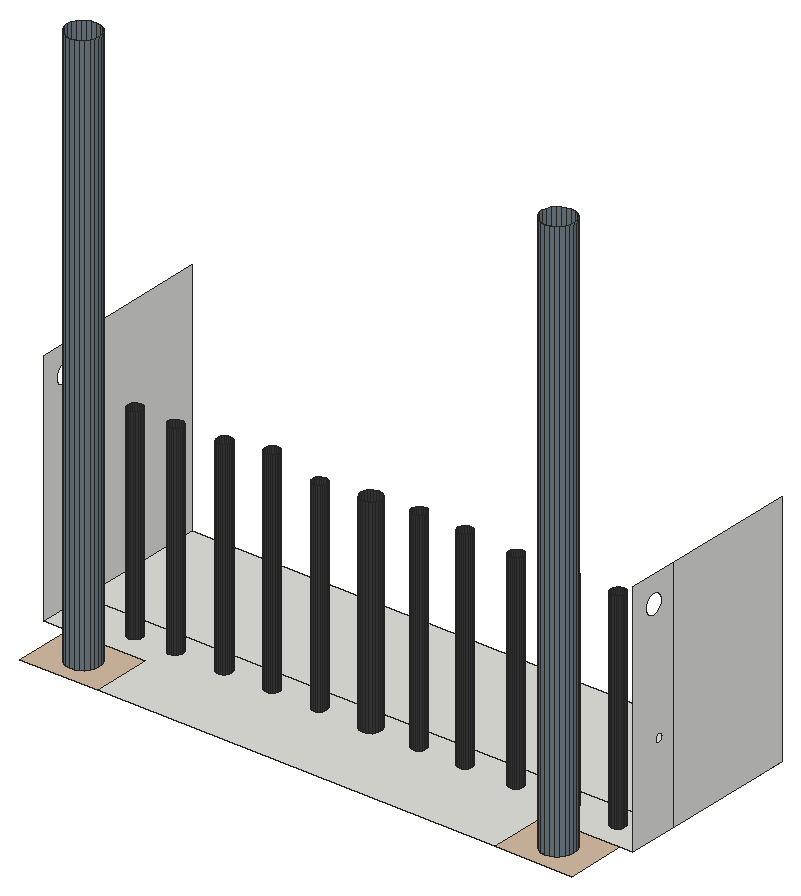
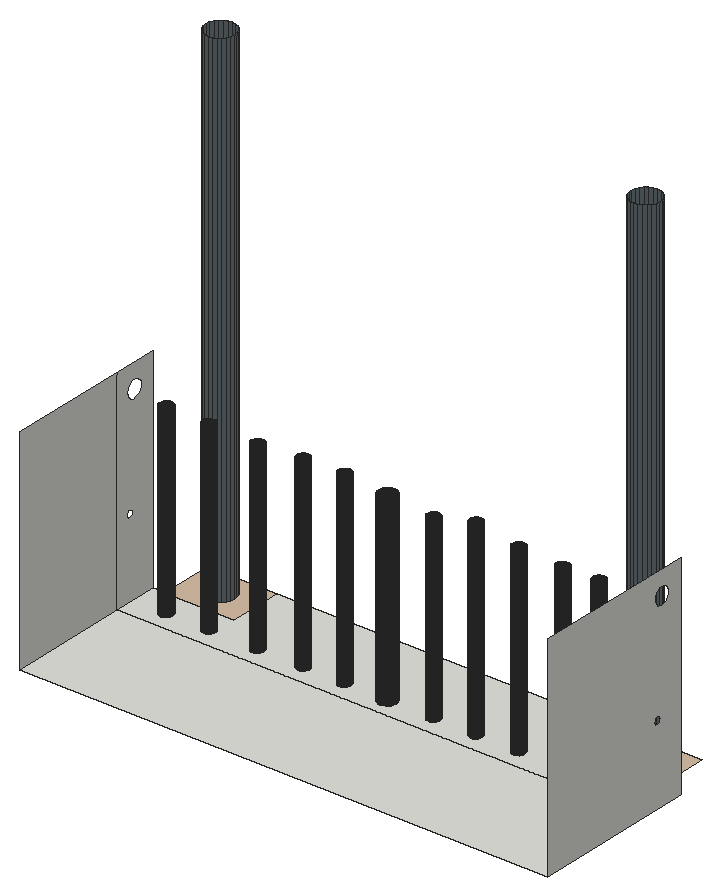
# SketchUp Ruby script. Lengths in inches.
U = 1.inch
M = Sketchup.active_model
def pt(a) = Geom::Point3d.new(a.map { |v| v * U })
def face(e, loops, mat)
  f = e.add_face(loops[0].map { |a| pt(a) })
  loops[1..].each { |l| e.add_face(l.map { |a| pt(a) }).erase! }
  f.material = f.back_material = mat if mat
  f
end
# faces: each face lists its corners as indices into pts; further lists are holes
def faces(e, pts, list, mat = nil) = list.each { |f| face(e, (f[0].is_a?(Array) ? f : [f]).map { |l| l.map { |i| pts[i] } }, mat) }
# xy, xz, yz: faces in a plane at the given z, y or x. An outline is a flat list of corners, or four numbers for a rectangle; further outlines are holes
def ring(l) = l.size == 4 ? [[l[0], l[1]], [l[2], l[1]], [l[2], l[3]], [l[0], l[3]]] : l.each_slice(2).to_a
def flat(e, list, mat, &to3) = list.each { |f| face(e, (f[0].is_a?(Array) ? f : [f]).map { |l| ring(l).map { |u, v| to3.(u, v) } }, mat) }
def xy(e, z, list, mat = nil) = flat(e, list, mat) { |x, y| [x, y, z] }
def xz(e, y, list, mat = nil) = flat(e, list, mat) { |x, z| [x, y, z] }
def yz(e, x, list, mat = nil) = flat(e, list, mat) { |y, z| [x, y, z] }
def lines(e, pts, list) = list.each { |a, b| e.add_line(pt(pts[a]), pt(pts[b])) }
# prism: a flat outline (further loops are holes) pulled along v
def prism(e, loops, v, mat = nil)
  f = face(e, loops, mat); d = Geom::Vector3d.new(v.map { |x| x * U })
  f.pushpull(f.normal.samedirection?(d) ? d.length : -d.length)
end
def box(e, o, s, mat = nil) = prism(e, [[o, [o[0] + s[0], o[1], o[2]], [o[0] + s[0], o[1] + s[1], o[2]], [o[0], o[1] + s[1], o[2]]]], [0, 0, s[2]], mat)
def at(x, y, z, deg = 0) = Geom::Transformation.translation(pt([x, y, z])) * Geom::Transformation.rotation(ORIGIN, Z_AXIS, deg.degrees)
def axes(o, x, y, z) = Geom::Transformation.new([*x, 0, *y, 0, *z, 0, *pt(o).to_a, 1])
def part(name) = M.definitions.add(name)
# library, detail: a bought-in or finely detailed component or shape, given as its bounding box
def library(name, o, s) = part(name).tap { |d| box(d.entities, o, s) }
def detail(e, o, s) = box(e.add_group.entities, o, s)
def put(e, d, t, mat = nil) = e.add_instance(d, t).tap { |i| i.material = mat if mat }
def group(e, t, mat = nil) = e.add_group.tap { |g| g.transformation = t; g.material = mat if mat }.entities
root = M.entities
M.materials.add("[Color M07]").color = [58, 58, 58]
M.materials.add("[Formica Laminate Light]").color = [213, 189, 164]
M.materials.add("[Formica Speckled Grey]").color = [112, 125, 132]
xy(root,162.85,[[[59.48,81.92,111.73,81.92,111.73,89.73,123.57,89.73,123.57,96.35,46.18,96.35,46.18,89.73,59.48,89.73],[86.23,92.1,85.89,92.15,85.57,92.28,85.3,92.48,85.09,92.76,84.96,93.07,84.92,93.41,84.96,93.75,85.09,94.07,85.3,94.34,85.57,94.55,85.89,94.68,86.23,94.73,86.57,94.68,86.89,94.55,87.16,94.34,87.37,94.07,87.5,93.75,87.54,93.41,87.5,93.07,87.37,92.76,87.16,92.48,86.89,92.28,86.57,92.15],[92.58,92.43,92.34,92.46,92.11,92.55,91.92,92.7,91.77,92.9,91.67,93.125,91.64,93.37,91.67,93.61,91.77,93.83,91.92,94.03,92.11,94.18,92.34,94.27,92.58,94.3,92.82,94.27,93.05,94.18,93.24,94.03,93.39,93.83,93.48,93.61,93.52,93.37,93.48,93.125,93.39,92.9,93.24,92.7,93.05,92.55,92.82,92.46],[98.64,92.43,98.4,92.46,98.17,92.55,97.98,92.7,97.83,92.9,97.74,93.125,97.7,93.37,97.74,93.61,97.83,93.83,97.98,94.03,98.17,94.18,98.4,94.27,98.64,94.3,98.88,94.27,99.11,94.18,99.3,94.03,99.45,93.83,99.55,93.61,99.58,93.37,99.55,93.125,99.45,92.9,99.3,92.7,99.11,92.55,98.88,92.46],[105.33,92.43,105.09,92.46,104.86,92.55,104.67,92.7,104.52,92.9,104.42,93.125,104.39,93.37,104.42,93.61,104.52,93.83,104.67,94.03,104.86,94.18,105.09,94.27,105.33,94.3,105.57,94.27,105.8,94.18,105.99,94.03,106.14,93.83,106.23,93.61,106.27,93.37,106.23,93.125,106.14,92.9,105.99,92.7,105.8,92.55,105.57,92.46],[112.45,92.43,112.21,92.46,111.99,92.55,111.79,92.7,111.64,92.9,111.55,93.125,111.52,93.37,111.55,93.61,111.64,93.83,111.79,94.03,111.99,94.18,112.21,94.27,112.45,94.3,112.7,94.27,112.92,94.18,113.12,94.03,113.27,93.83,113.36,93.61,113.39,93.37,113.36,93.125,113.27,92.9,113.12,92.7,112.92,92.55,112.7,92.46],[79.52,92.43,79.27,92.46,79.05,92.55,78.85,92.7,78.7,92.9,78.61,93.125,78.58,93.37,78.61,93.61,78.7,93.83,78.85,94.03,79.05,94.18,79.27,94.27,79.52,94.3,79.76,94.27,79.99,94.18,80.18,94.03,80.33,93.83,80.42,93.61,80.45,93.37,80.42,93.125,80.33,92.9,80.18,92.7,79.99,92.55,79.76,92.46],[49.7,92.43,49.46,92.46,49.24,92.55,49.04,92.7,48.89,92.9,48.8,93.125,48.77,93.37,48.8,93.61,48.89,93.83,49.04,94.03,49.24,94.18,49.46,94.27,49.7,94.3,49.95,94.27,50.17,94.18,50.37,94.03,50.52,93.83,50.61,93.61,50.64,93.37,50.61,93.125,50.52,92.9,50.37,92.7,50.17,92.55,49.95,92.46],[73.27,92.43,73.02,92.46,72.8,92.55,72.6,92.7,72.45,92.9,72.36,93.125,72.33,93.37,72.36,93.61,72.45,93.83,72.6,94.03,72.8,94.18,73.02,94.27,73.27,94.3,73.51,94.27,73.74,94.18,73.93,94.03,74.08,93.83,74.17,93.61,74.2,93.37,74.17,93.125,74.08,92.9,73.93,92.7,73.74,92.55,73.51,92.46],[55.27,92.43,55.02,92.46,54.8,92.55,54.6,92.7,54.45,92.9,54.36,93.125,54.33,93.37,54.36,93.61,54.45,93.83,54.6,94.03,54.8,94.18,55.02,94.27,55.27,94.3,55.51,94.27,55.74,94.18,55.93,94.03,56.08,93.83,56.17,93.61,56.2,93.37,56.17,93.125,56.08,92.9,55.93,92.7,55.74,92.55,55.51,92.46],[67.02,92.43,66.77,92.46,66.55,92.55,66.35,92.7,66.2,92.9,66.11,93.125,66.08,93.37,66.11,93.61,66.2,93.83,66.35,94.03,66.55,94.18,66.77,94.27,67.02,94.3,67.26,94.27,67.49,94.18,67.68,94.03,67.83,93.83,67.92,93.61,67.95,93.37,67.92,93.125,67.83,92.9,67.68,92.7,67.49,92.55,67.26,92.46],[60.58,92.43,60.34,92.46,60.11,92.55,59.92,92.7,59.77,92.9,59.67,93.125,59.64,93.37,59.67,93.61,59.77,93.83,59.92,94.03,60.11,94.18,60.34,94.27,60.58,94.3,60.82,94.27,61.05,94.18,61.24,94.03,61.39,93.83,61.48,93.61,61.52,93.37,61.48,93.125,61.39,92.9,61.24,92.7,61.05,92.55,60.82,92.46],[118.7,92.43,118.46,92.46,118.24,92.55,118.04,92.7,117.89,92.9,117.8,93.125,117.77,93.37,117.8,93.61,117.89,93.83,118.04,94.03,118.24,94.18,118.46,94.27,118.7,94.3,118.95,94.27,119.17,94.18,119.37,94.03,119.52,93.83,119.61,93.61,119.64,93.37,119.61,93.125,119.52,92.9,119.37,92.7,119.17,92.55,118.95,92.46]],[54.42,83.75,53.87,83.82,53.36,84.04,52.92,84.375,52.58,84.81,52.37,85.33,52.3,85.88,52.37,86.43,52.58,86.94,52.92,87.38,53.36,87.72,53.87,87.93,54.42,88,54.97,87.93,55.49,87.72,55.93,87.38,56.26,86.94,56.48,86.43,56.55,85.88,56.48,85.33,56.26,84.81,55.93,84.375,55.49,84.04,54.97,83.82],[116.8,83.75,116.25,83.82,115.74,84.04,115.3,84.375,114.96,84.81,114.75,85.33,114.67,85.88,114.75,86.43,114.96,86.94,115.3,87.38,115.74,87.72,116.25,87.93,116.8,88,117.35,87.93,117.86,87.72,118.3,87.38,118.64,86.94,118.85,86.43,118.92,85.88,118.85,85.33,118.64,84.81,118.3,84.375,117.86,84.04,117.35,83.82],[49.7,92.43,49.46,92.46,49.24,92.55,49.04,92.7,48.89,92.9,48.8,93.125,48.77,93.37,48.8,93.61,48.89,93.83,49.04,94.03,49.24,94.18,49.46,94.27,49.7,94.3,49.95,94.27,50.17,94.18,50.37,94.03,50.52,93.83,50.61,93.61,50.64,93.37,50.61,93.125,50.52,92.9,50.37,92.7,50.17,92.55,49.95,92.46],[55.27,92.43,55.02,92.46,54.8,92.55,54.6,92.7,54.45,92.9,54.36,93.125,54.33,93.37,54.36,93.61,54.45,93.83,54.6,94.03,54.8,94.18,55.02,94.27,55.27,94.3,55.51,94.27,55.74,94.18,55.93,94.03,56.08,93.83,56.17,93.61,56.2,93.37,56.17,93.125,56.08,92.9,55.93,92.7,55.74,92.55,55.51,92.46],
  [60.58,92.43,60.34,92.46,60.11,92.55,59.92,92.7,59.77,92.9,59.67,93.125,59.64,93.37,59.67,93.61,59.77,93.83,59.92,94.03,60.11,94.18,60.34,94.27,60.58,94.3,60.82,94.27,61.05,94.18,61.24,94.03,61.39,93.83,61.48,93.61,61.52,93.37,61.48,93.125,61.39,92.9,61.24,92.7,61.05,92.55,60.82,92.46],[67.02,92.43,66.77,92.46,66.55,92.55,66.35,92.7,66.2,92.9,66.11,93.125,66.08,93.37,66.11,93.61,66.2,93.83,66.35,94.03,66.55,94.18,66.77,94.27,67.02,94.3,67.26,94.27,67.49,94.18,67.68,94.03,67.83,93.83,67.92,93.61,67.95,93.37,67.92,93.125,67.83,92.9,67.68,92.7,67.49,92.55,67.26,92.46],[73.27,92.43,73.02,92.46,72.8,92.55,72.6,92.7,72.45,92.9,72.36,93.125,72.33,93.37,72.36,93.61,72.45,93.83,72.6,94.03,72.8,94.18,73.02,94.27,73.27,94.3,73.51,94.27,73.74,94.18,73.93,94.03,74.08,93.83,74.17,93.61,74.2,93.37,74.17,93.125,74.08,92.9,73.93,92.7,73.74,92.55,73.51,92.46],[79.52,92.43,79.27,92.46,79.05,92.55,78.85,92.7,78.7,92.9,78.61,93.125,78.58,93.37,78.61,93.61,78.7,93.83,78.85,94.03,79.05,94.18,79.27,94.27,79.52,94.3,79.76,94.27,79.99,94.18,80.18,94.03,80.33,93.83,80.42,93.61,80.45,93.37,80.42,93.125,80.33,92.9,80.18,92.7,79.99,92.55,79.76,92.46],[92.58,92.43,92.34,92.46,92.11,92.55,91.92,92.7,91.77,92.9,91.67,93.125,91.64,93.37,91.67,93.61,91.77,93.83,91.92,94.03,92.11,94.18,92.34,94.27,92.58,94.3,92.82,94.27,93.05,94.18,93.24,94.03,93.39,93.83,93.48,93.61,93.52,93.37,93.48,93.125,93.39,92.9,93.24,92.7,93.05,92.55,92.82,92.46],
  [98.64,92.43,98.4,92.46,98.17,92.55,97.98,92.7,97.83,92.9,97.74,93.125,97.7,93.37,97.74,93.61,97.83,93.83,97.98,94.03,98.17,94.18,98.4,94.27,98.64,94.3,98.88,94.27,99.11,94.18,99.3,94.03,99.45,93.83,99.55,93.61,99.58,93.37,99.55,93.125,99.45,92.9,99.3,92.7,99.11,92.55,98.88,92.46],[105.33,92.43,105.09,92.46,104.86,92.55,104.67,92.7,104.52,92.9,104.42,93.125,104.39,93.37,104.42,93.61,104.52,93.83,104.67,94.03,104.86,94.18,105.09,94.27,105.33,94.3,105.57,94.27,105.8,94.18,105.99,94.03,106.14,93.83,106.23,93.61,106.27,93.37,106.23,93.125,106.14,92.9,105.99,92.7,105.8,92.55,105.57,92.46],[112.45,92.43,112.21,92.46,111.99,92.55,111.79,92.7,111.64,92.9,111.55,93.125,111.52,93.37,111.55,93.61,111.64,93.83,111.79,94.03,111.99,94.18,112.21,94.27,112.45,94.3,112.7,94.27,112.92,94.18,113.12,94.03,113.27,93.83,113.36,93.61,113.39,93.37,113.36,93.125,113.27,92.9,113.12,92.7,112.92,92.55,112.7,92.46],[118.7,92.43,118.46,92.46,118.24,92.55,118.04,92.7,117.89,92.9,117.8,93.125,117.77,93.37,117.8,93.61,117.89,93.83,118.04,94.03,118.24,94.18,118.46,94.27,118.7,94.3,118.95,94.27,119.17,94.18,119.37,94.03,119.52,93.83,119.61,93.61,119.64,93.37,119.61,93.125,119.52,92.9,119.37,92.7,119.17,92.55,118.95,92.46],[46.18,96.35,123.57,114.1]])
xy(root,162.85,[[[49.36,81.92,59.48,89.73],[54.42,83.75,53.87,83.82,53.36,84.04,52.92,84.375,52.58,84.81,52.37,85.33,52.3,85.88,52.37,86.43,52.58,86.94,52.92,87.38,53.36,87.72,53.87,87.93,54.42,88,54.97,87.93,55.49,87.72,55.93,87.38,56.26,86.94,56.48,86.43,56.55,85.88,56.48,85.33,56.26,84.81,55.93,84.375,55.49,84.04,54.97,83.82]],[[111.73,81.92,121.85,89.73],[116.8,83.75,116.25,83.82,115.74,84.04,115.3,84.375,114.96,84.81,114.75,85.33,114.67,85.88,114.75,86.43,114.96,86.94,115.3,87.38,115.74,87.72,116.25,87.93,116.8,88,117.35,87.93,117.86,87.72,118.3,87.38,118.64,86.94,118.85,86.43,118.92,85.88,118.85,85.33,118.64,84.81,118.3,84.375,117.86,84.04,117.35,83.82]]],"[Formica Laminate Light]")
yz(root,46.18,[[[89.73,162.85,114.1,194.03],[93.14,189.23,92.8,189.28,92.48,189.41,92.21,189.62,92,189.89,91.87,190.21,91.82,190.55,91.87,190.89,92,191.2,92.21,191.47,92.48,191.68,92.8,191.81,93.14,191.86,93.48,191.81,93.79,191.68,94.06,191.47,94.27,191.2,94.4,190.89,94.45,190.55,94.4,190.21,94.27,189.89,94.06,189.62,93.79,189.41,93.48,189.28],[94.01,173.9,93.86,173.92,93.73,173.98,93.61,174.07,93.52,174.18,93.47,174.32,93.45,174.47,93.47,174.61,93.52,174.75,93.61,174.86,93.73,174.95,93.86,175.01,94.01,175.03,94.15,175.01,94.29,174.95,94.41,174.86,94.5,174.75,94.55,174.61,94.57,174.47,94.55,174.32,94.5,174.18,94.41,174.07,94.29,173.98,94.15,173.92]]])
yz(root,123.57,[[[89.73,162.85,96.35,194.03],[93.14,189.23,93.48,189.28,93.79,189.41,94.06,189.62,94.27,189.89,94.4,190.21,94.45,190.55,94.4,190.89,94.27,191.2,94.06,191.47,93.79,191.68,93.48,191.81,93.14,191.86,92.8,191.81,92.48,191.68,92.21,191.47,92,191.2,91.87,190.89,91.82,190.55,91.87,190.21,92,189.89,92.21,189.62,92.48,189.41,92.8,189.28],[94.01,173.9,94.15,173.92,94.29,173.98,94.41,174.07,94.5,174.18,94.55,174.32,94.57,174.47,94.55,174.61,94.5,174.75,94.41,174.86,94.29,174.95,94.15,175.01,94.01,175.03,93.86,175.01,93.73,174.95,93.61,174.86,93.52,174.75,93.47,174.61,93.45,174.47,93.47,174.32,93.52,174.18,93.61,174.07,93.73,173.98,93.86,173.92]],[96.35,162.85,114.1,194.03]])
p = [[53.36,84.04,162.85],[53.87,83.82,162.85],[53.87,83.82,236.95],[53.36,84.04,236.95],[54.42,83.75,162.85],[54.42,83.75,236.95],
  [54.97,83.82,162.85],[54.97,83.82,236.95],[55.49,84.04,162.85],[55.49,84.04,236.95],[115.74,84.04,162.85],[116.25,83.82,162.85],
  [116.25,83.82,236.95],[115.74,84.04,236.95],[116.8,83.75,162.85],[116.8,83.75,236.95],[117.35,83.82,162.85],[117.35,83.82,236.95],
  [117.86,84.04,162.85],[117.86,84.04,236.95],[52.92,84.375,162.85],[52.92,84.375,236.95],[55.93,84.375,162.85],[55.93,84.375,236.95],
  [115.3,84.375,162.85],[115.3,84.375,236.95],[118.3,84.375,162.85],[118.3,84.375,236.95],[52.58,84.81,162.85],[52.58,84.81,236.95],
  [56.26,84.81,162.85],[56.26,84.81,236.95],[114.96,84.81,162.85],[114.96,84.81,236.95],[118.64,84.81,162.85],[118.64,84.81,236.95],
  [52.37,85.33,162.85],[52.37,85.33,236.95],[56.48,85.33,162.85],[56.48,85.33,236.95],[114.75,85.33,162.85],[114.75,85.33,236.95],
  [118.85,85.33,162.85],[118.85,85.33,236.95],[52.3,85.88,162.85],[52.3,85.88,236.95],[56.55,85.88,162.85],[56.55,85.88,236.95],
  [114.67,85.88,162.85],[114.67,85.88,236.95],[118.92,85.88,162.85],[118.92,85.88,236.95],[52.37,86.43,162.85],[52.37,86.43,236.95],
  [56.48,86.43,162.85],[56.48,86.43,236.95],[114.75,86.43,162.85],[114.75,86.43,236.95],[118.85,86.43,162.85],[118.85,86.43,236.95],
  [52.58,86.94,162.85],[52.58,86.94,236.95],[56.26,86.94,162.85],[56.26,86.94,236.95],[114.96,86.94,162.85],[114.96,86.94,236.95],
  [118.64,86.94,162.85],[118.64,86.94,236.95],[52.92,87.38,162.85],[52.92,87.38,236.95],[55.93,87.38,162.85],[55.93,87.38,236.95],
  [115.3,87.38,162.85],[115.3,87.38,236.95],[118.3,87.38,162.85],[118.3,87.38,236.95],[53.36,87.72,162.85],[53.36,87.72,236.95],
  [55.49,87.72,162.85],[55.49,87.72,236.95],[115.74,87.72,162.85],[115.74,87.72,236.95],[117.86,87.72,162.85],[117.86,87.72,236.95],
  [53.87,87.93,162.85],[53.87,87.93,236.95],[54.97,87.93,162.85],[54.97,87.93,236.95],[116.25,87.93,162.85],[116.25,87.93,236.95],
  [117.35,87.93,162.85],[117.35,87.93,236.95],[54.42,88,162.85],[54.42,88,236.95],[116.8,88,162.85],[116.8,88,236.95],
  [85.57,92.28,162.85],[85.89,92.15,162.85],[85.89,92.15,190.03],[85.57,92.28,190.03],[86.23,92.1,162.85],[86.23,92.1,190.03],
  [86.57,92.15,162.85],[86.57,92.15,190.03],[86.89,92.28,162.85],[86.89,92.28,190.03],[85.3,92.48,162.85],[85.3,92.48,190.03],
  [87.16,92.48,162.85],[87.16,92.48,190.03],[49.46,92.46,162.85],[49.7,92.43,162.85],[49.7,92.43,189.85],[49.46,92.46,189.85],
  [49.95,92.46,162.85],[49.95,92.46,189.85],[55.02,92.46,162.85],[55.27,92.43,162.85],[55.27,92.43,189.6],[55.02,92.46,189.6],
  [55.51,92.46,162.85],[55.51,92.46,189.6],[60.34,92.46,162.85],[60.58,92.43,162.85],[60.58,92.43,189.53],[60.34,92.46,189.53],
  [60.82,92.46,162.85],[60.82,92.46,189.53],[66.77,92.46,162.85],[67.02,92.43,162.85],[67.02,92.43,189.85],[66.77,92.46,189.85],
  [67.26,92.46,162.85],[67.26,92.46,189.85],[73.02,92.46,162.85],[73.27,92.43,162.85],[73.27,92.43,190.89],[73.02,92.46,190.89],
  [73.51,92.46,162.85],[73.51,92.46,190.89],[79.27,92.46,162.85],[79.52,92.43,162.85],[79.52,92.43,189.41],[79.27,92.46,189.41],
  [79.76,92.46,162.85],[79.76,92.46,189.41],[92.34,92.46,162.85],[92.58,92.43,162.85],[92.58,92.43,190.53],[92.34,92.46,190.53],
  [92.82,92.46,162.85],[92.82,92.46,190.53],[98.4,92.46,162.85],[98.64,92.43,162.85],[98.64,92.43,190.41],[98.4,92.46,190.41],
  [98.88,92.46,162.85],[98.88,92.46,190.41],[105.09,92.46,162.85],[105.33,92.43,162.85],[105.33,92.43,189.97],[105.09,92.46,189.97],
  [105.57,92.46,162.85],[105.57,92.46,189.97],[112.21,92.46,162.85],[112.45,92.43,162.85],[112.45,92.43,190.1],[112.21,92.46,190.1],
  [112.7,92.46,162.85],[112.7,92.46,190.1],[118.46,92.46,162.85],[118.7,92.43,162.85],[118.7,92.43,190.22],[118.46,92.46,190.22],
  [118.95,92.46,162.85],[118.95,92.46,190.22],[49.24,92.55,162.85],[49.24,92.55,189.85],[50.17,92.55,162.85],[50.17,92.55,189.85],
  [54.8,92.55,162.85],[54.8,92.55,189.6],[55.74,92.55,162.85],[55.74,92.55,189.6],[60.11,92.55,162.85],[60.11,92.55,189.53],
  [61.05,92.55,162.85],[61.05,92.55,189.53],[66.55,92.55,162.85],[66.55,92.55,189.85],[67.49,92.55,162.85],[67.49,92.55,189.85],
  [72.8,92.55,162.85],[72.8,92.55,190.89],[73.74,92.55,162.85],[73.74,92.55,190.89],[79.05,92.55,162.85],[79.23,92.48,189.41],
  [79.05,92.55,189.41],[79.99,92.55,162.85],[79.99,92.55,189.41],[79.81,92.48,189.41],[85.09,92.76,162.85],[85.09,92.76,190.03],
  [87.37,92.76,162.85],[87.37,92.76,190.03],[92.11,92.55,162.85],[92.11,92.55,190.53],[93.05,92.55,162.85],[93.05,92.55,190.53],
  [98.17,92.55,162.85],[98.17,92.55,190.41],[99.11,92.55,162.85],[99.11,92.55,190.41],[104.86,92.55,162.85],[104.86,92.55,189.97],
  [105.8,92.55,162.85],[105.8,92.55,189.97],[111.99,92.55,162.85],[111.99,92.55,190.1],[112.92,92.55,162.85],[112.92,92.55,190.1],
  [118.24,92.55,162.85],[118.24,92.55,190.22],[119.17,92.55,162.85],[119.17,92.55,190.22],[49.04,92.7,162.85],[49.04,92.7,189.85],
  [50.37,92.7,162.85],[50.37,92.7,189.85],[54.6,92.7,162.85],[54.6,92.7,189.6],[55.93,92.7,162.85],[55.93,92.7,189.6],
  [59.92,92.7,162.85],[59.92,92.7,189.53],[61.24,92.7,162.85],[61.24,92.7,189.53],[66.35,92.7,162.85],[66.35,92.7,189.85],
  [67.68,92.7,162.85],[67.68,92.7,189.85],[72.6,92.7,162.85],[72.6,92.7,190.89],[73.93,92.7,162.85],[73.93,92.7,190.89],
  [78.85,92.7,162.85],[78.85,92.7,189.41],[80.18,92.7,162.85],[80.18,92.7,189.41],[91.92,92.7,162.85],[91.92,92.7,190.53],
  [93.24,92.7,162.85],[93.24,92.7,190.53],[97.98,92.7,162.85],[97.98,92.7,190.41],[99.3,92.7,162.85],[99.3,92.7,190.41],
  [104.67,92.7,162.85],[104.67,92.7,189.97],[105.99,92.7,162.85],[105.99,92.7,189.97],[111.79,92.7,162.85],[111.79,92.7,190.1],
  [113.12,92.7,162.85],[113.12,92.7,190.1],[118.04,92.7,162.85],[118.04,92.7,190.22],[119.37,92.7,162.85],[119.37,92.7,190.22],
  [48.89,92.9,162.85],[48.89,92.9,189.85],[50.52,92.9,162.85],[50.52,92.9,189.85],[54.45,92.9,162.85],[54.45,92.9,189.6],
  [56.08,92.9,162.85],[56.08,92.9,189.6],[59.77,92.9,162.85],[59.77,92.9,189.53],[61.39,92.9,162.85],[61.39,92.9,189.53],
  [66.2,92.9,162.85],[66.2,92.9,189.85],[67.83,92.9,162.85],[67.83,92.9,189.85],[72.45,92.9,162.85],[72.45,92.9,190.89],
  [74.08,92.9,162.85],[74.08,92.9,190.89],[78.7,92.9,162.85],[78.7,92.9,189.41],[80.33,92.9,162.85],[80.33,92.9,189.41],
  [91.77,92.9,162.85],[91.77,92.9,190.53],[93.39,92.9,162.85],[93.39,92.9,190.53],[97.83,92.9,162.85],[97.83,92.9,190.41],
  [99.45,92.9,162.85],[99.45,92.9,190.41],[104.52,92.9,162.85],[104.52,92.9,189.97],[106.14,92.9,162.85],[106.14,92.9,189.97],
  [111.64,92.9,162.85],[111.64,92.9,190.1],[113.27,92.9,162.85],[113.27,92.9,190.1],[117.89,92.9,162.85],[117.89,92.9,190.22],
  [119.52,92.9,162.85],[119.52,92.9,190.22],[84.96,93.07,162.85],[84.96,93.07,190.03],[87.5,93.07,162.85],[87.5,93.07,190.03],
  [48.8,93.125,162.85],[48.8,93.125,189.85],[50.61,93.125,162.85],[50.61,93.125,189.85],[54.36,93.125,162.85],[54.36,93.125,189.6],
  [56.17,93.125,162.85],[56.17,93.125,189.6],[59.67,93.125,162.85],[59.67,93.125,189.53],[61.48,93.125,162.85],[61.48,93.125,189.53],
  [66.11,93.125,162.85],[66.11,93.125,189.85],[67.92,93.125,162.85],[67.92,93.125,189.85],[72.36,93.125,162.85],[72.36,93.125,190.89],
  [74.17,93.125,162.85],[74.17,93.125,190.89],[78.61,93.125,162.85],[78.61,93.125,189.41],[80.42,93.125,162.85],[80.42,93.125,189.41],
  [91.67,93.125,162.85],[91.67,93.125,190.53],[93.48,93.125,162.85],[93.48,93.125,190.53],[97.74,93.125,162.85],[97.74,93.125,190.41],
  [99.55,93.125,162.85],[99.55,93.125,190.41],[104.42,93.125,162.85],[104.42,93.125,189.97],[106.23,93.125,162.85],[106.23,93.125,189.97],
  [111.55,93.125,162.85],[111.55,93.125,190.1],[113.36,93.125,162.85],[113.36,93.125,190.1],[117.8,93.125,162.85],[117.8,93.125,190.22],
  [119.61,93.125,162.85],[119.61,93.125,190.22],[48.77,93.37,162.85],[48.77,93.37,189.85],[50.64,93.37,162.85],[50.64,93.37,189.85],
  [54.33,93.37,162.85],[54.33,93.37,189.6],[56.2,93.37,162.85],[56.2,93.37,189.6],[59.64,93.37,162.85],[59.64,93.37,189.53],
  [61.52,93.37,162.85],[61.52,93.37,189.53],[66.08,93.37,162.85],[66.08,93.37,189.85],[67.95,93.37,162.85],[67.95,93.37,189.85],
  [72.33,93.37,162.85],[72.33,93.37,190.89],[74.2,93.37,162.85],[74.2,93.37,190.89],[78.58,93.37,162.85],[78.58,93.37,189.41],
  [80.45,93.37,162.85],[80.45,93.37,189.41],[84.92,93.41,162.85],[84.92,93.41,190.03],[87.54,93.41,162.85],[87.54,93.41,190.03],
  [91.64,93.37,162.85],[91.64,93.37,190.53],[93.52,93.37,162.85],[93.52,93.37,190.53],[97.7,93.37,162.85],[97.7,93.37,190.41],
  [99.58,93.37,162.85],[99.58,93.37,190.41],[104.39,93.37,162.85],[104.39,93.37,189.97],[106.27,93.37,162.85],[106.27,93.37,189.97],
  [111.52,93.37,162.85],[111.52,93.37,190.1],[113.39,93.37,162.85],[113.39,93.37,190.1],[117.77,93.37,162.85],[117.77,93.37,190.22],
  [119.64,93.37,162.85],[119.64,93.37,190.22],[48.8,93.61,162.85],[48.8,93.61,189.85],[50.61,93.61,162.85],[50.61,93.61,189.85],
  [54.36,93.61,162.85],[54.36,93.61,189.6],[56.17,93.61,162.85],[56.17,93.61,189.6],[59.67,93.61,162.85],[59.67,93.61,189.53],
  [61.48,93.61,162.85],[61.48,93.61,189.53],[66.11,93.61,162.85],[66.11,93.61,189.85],[67.92,93.61,162.85],[67.92,93.61,189.85],
  [72.36,93.61,162.85],[72.36,93.61,190.89],[74.17,93.61,162.85],[74.17,93.61,190.89],[78.61,93.61,162.85],[78.61,93.61,189.41],
  [80.42,93.61,162.85],[80.42,93.61,189.41],[84.96,93.75,162.85],[84.96,93.75,190.03],[87.5,93.75,162.85],[87.5,93.75,190.03],
  [91.67,93.61,162.85],[91.67,93.61,190.53],[93.48,93.61,162.85],[93.48,93.61,190.53],[97.74,93.61,162.85],[97.74,93.61,190.41],
  [99.55,93.61,162.85],[99.55,93.61,190.41],[104.42,93.61,162.85],[104.42,93.61,189.97],[106.23,93.61,162.85],[106.23,93.61,189.97],
  [111.55,93.61,162.85],[111.55,93.61,190.1],[113.36,93.61,162.85],[113.36,93.61,190.1],[117.8,93.61,162.85],[117.8,93.61,190.22],
  [119.61,93.61,162.85],[119.61,93.61,190.22],[48.89,93.83,162.85],[48.89,93.83,189.85],[50.52,93.83,162.85],[50.52,93.83,189.85],
  [54.45,93.83,162.85],[54.45,93.83,189.6],[56.08,93.83,162.85],[56.08,93.83,189.6],[59.77,93.83,162.85],[59.77,93.83,189.53],
  [61.39,93.83,162.85],[61.39,93.83,189.53],[66.2,93.83,162.85],[66.2,93.83,189.85],[67.83,93.83,162.85],[67.83,93.83,189.85],
  [72.45,93.83,162.85],[72.45,93.83,190.89],[74.08,93.83,162.85],[74.08,93.83,190.89],[78.7,93.83,162.85],[78.6875,93.79,189.41],
  [78.7,93.83,189.41],[80.33,93.83,162.85],[80.33,93.83,189.41],[80.35,93.79,189.41],[91.77,93.83,162.85],[91.77,93.83,190.53],
  [93.39,93.83,162.85],[93.39,93.83,190.53],[97.83,93.83,162.85],[97.83,93.83,190.41],[99.45,93.83,162.85],[99.45,93.83,190.41],
  [104.52,93.83,162.85],[104.52,93.83,189.97],[106.14,93.83,162.85],[106.14,93.83,189.97],[111.64,93.83,162.85],[111.64,93.83,190.1],
  [113.27,93.83,162.85],[113.27,93.83,190.1],[117.89,93.83,162.85],[117.89,93.83,190.22],[119.52,93.83,162.85],[119.52,93.83,190.22],
  [49.04,94.03,162.85],[49.04,94.03,189.85],[50.37,94.03,162.85],[50.37,94.03,189.85],[54.6,94.03,162.85],[54.6,94.03,189.6],
  [55.93,94.03,162.85],[55.93,94.03,189.6],[59.92,94.03,162.85],[59.92,94.03,189.53],[61.24,94.03,162.85],[61.24,94.03,189.53],
  [66.35,94.03,162.85],[66.35,94.03,189.85],[67.68,94.03,162.85],[67.68,94.03,189.85],[72.6,94.03,162.85],[72.6,94.03,190.89],
  [73.93,94.03,162.85],[73.93,94.03,190.89],[78.85,94.03,162.85],[78.85,94.03,189.41],[80.18,94.03,162.85],[80.18,94.03,189.41],
  [85.09,94.07,162.85],[85.09,94.07,190.03],[87.37,94.07,162.85],[87.37,94.07,190.03],[91.92,94.03,162.85],[91.92,94.03,190.53],
  [93.24,94.03,162.85],[93.24,94.03,190.53],[97.98,94.03,162.85],[97.98,94.03,190.41],[99.3,94.03,162.85],[99.3,94.03,190.41],
  [104.67,94.03,162.85],[104.67,94.03,189.97],[105.99,94.03,162.85],[105.99,94.03,189.97],[111.79,94.03,162.85],[111.79,94.03,190.1],
  [113.12,94.03,162.85],[113.12,94.03,190.1],[118.04,94.03,162.85],[118.04,94.03,190.22],[119.37,94.03,162.85],[119.37,94.03,190.22],
  [49.24,94.18,162.85],[49.24,94.18,189.85],[50.17,94.18,162.85],[50.17,94.18,189.85],[54.8,94.18,162.85],[54.8,94.18,189.6],
  [55.74,94.18,162.85],[55.74,94.18,189.6],[60.11,94.18,162.85],[60.11,94.18,189.53],[61.05,94.18,162.85],[61.05,94.18,189.53],
  [66.55,94.18,162.85],[66.55,94.18,189.85],[67.49,94.18,162.85],[67.49,94.18,189.85],[72.8,94.18,162.85],[72.8,94.18,190.89],
  [73.74,94.18,162.85],[73.74,94.18,190.89],[79.05,94.18,162.85],[79.05,94.18,189.41],[79.99,94.18,162.85],[79.99,94.18,189.41],
  [92.11,94.18,162.85],[92.11,94.18,190.53],[93.05,94.18,162.85],[93.05,94.18,190.53],[98.17,94.18,162.85],[98.17,94.18,190.41],
  [99.11,94.18,162.85],[99.11,94.18,190.41],[104.86,94.18,162.85],[104.86,94.18,189.97],[105.8,94.18,162.85],[105.8,94.18,189.97],
  [111.99,94.18,162.85],[111.99,94.18,190.1],[112.92,94.18,162.85],[112.92,94.18,190.1],[118.24,94.18,162.85],[118.24,94.18,190.22],
  [119.17,94.18,162.85],[119.17,94.18,190.22],[85.3,94.34,162.85],[85.3,94.34,190.03],[87.16,94.34,162.85],[87.16,94.34,190.03],
  [49.46,94.27,162.85],[49.46,94.27,189.85],[49.95,94.27,162.85],[49.95,94.27,189.85],[55.02,94.27,162.85],[55.02,94.27,189.6],
  [55.51,94.27,162.85],[55.51,94.27,189.6],[60.34,94.27,162.85],[60.34,94.27,189.53],[60.82,94.27,162.85],[60.82,94.27,189.53],
  [66.77,94.27,162.85],[66.77,94.27,189.85],[67.26,94.27,162.85],[67.26,94.27,189.85],[73.02,94.27,162.85],[73.02,94.27,190.89],
  [73.51,94.27,162.85],[73.51,94.27,190.89],[79.27,94.27,162.85],[79.27,94.27,189.41],[79.76,94.27,162.85],[79.76,94.27,189.41],
  [92.34,94.27,162.85],[92.34,94.27,190.53],[92.82,94.27,162.85],[92.82,94.27,190.53],[98.4,94.27,162.85],[98.4,94.27,190.41],
  [98.88,94.27,162.85],[98.88,94.27,190.41],[105.09,94.27,162.85],[105.09,94.27,189.97],[105.57,94.27,162.85],[105.57,94.27,189.97],
  [112.21,94.27,162.85],[112.21,94.27,190.1],[112.7,94.27,162.85],[112.7,94.27,190.1],[118.46,94.27,162.85],[118.46,94.27,190.22],
  [118.95,94.27,162.85],[118.95,94.27,190.22],[49.7,94.3,162.85],[49.7,94.3,189.85],[55.27,94.3,162.85],[55.27,94.3,189.6],
  [60.58,94.3,162.85],[60.58,94.3,189.53],[67.02,94.3,162.85],[67.02,94.3,189.85],[73.27,94.3,162.85],[73.27,94.3,190.89],
  [79.52,94.3,162.85],[79.52,94.3,189.41],[85.57,94.55,162.85],[85.57,94.55,190.03],[86.89,94.55,162.85],[86.89,94.55,190.03],
  [92.58,94.3,162.85],[92.58,94.3,190.53],[98.64,94.3,162.85],[98.64,94.3,190.41],[105.33,94.3,162.85],[105.33,94.3,189.97],
  [112.45,94.3,162.85],[112.45,94.3,190.1],[118.7,94.3,162.85],[118.7,94.3,190.22],[85.89,94.68,162.85],[85.89,94.68,190.03],
  [86.57,94.68,162.85],[86.57,94.68,190.03],[86.23,94.73,162.85],[86.23,94.73,190.03]]
faces(root,p,[[0,1,2,3],[1,4,5,2],[4,6,7,5],[6,8,9,7],[10,11,12,13],[11,14,15,12],[14,16,17,15],[16,18,19,17],
  [20,0,3,21],[8,22,23,9],[24,10,13,25],[18,26,27,19],[28,20,21,29],[22,30,31,23],[32,24,25,33],[26,34,35,27],
  [36,28,29,37],[30,38,39,31],[40,32,33,41],[34,42,43,35],[44,36,37,45],[38,46,47,39],[48,40,41,49],[42,50,51,43],
  [52,44,45,53],[46,54,55,47],[56,48,49,57],[50,58,59,51],[60,52,53,61],[54,62,63,55],[64,56,57,65],[58,66,67,59],
  [68,60,61,69],[62,70,71,63],[72,64,65,73],[66,74,75,67],[76,68,69,77],[70,78,79,71],[80,72,73,81],[74,82,83,75],
  [84,76,77,85],[78,86,87,79],[88,80,81,89],[82,90,91,83],[92,84,85,93],[86,92,93,87],[94,88,89,95],[90,94,95,91]],"[Formica Speckled Grey]")
faces(root,p,[[96,97,98,99],[97,100,101,98],[100,102,103,101],[102,104,105,103],[106,96,99,107],[104,108,109,105],[110,111,112,113],[111,114,115,112],
  [116,117,118,119],[117,120,121,118],[122,123,124,125],[123,126,127,124],[128,129,130,131],[129,132,133,130],[134,135,136,137],[135,138,139,136],
  [140,141,142,143],[141,144,145,142],[146,147,148,149],[147,150,151,148],[152,153,154,155],[153,156,157,154],[158,159,160,161],[159,162,163,160],
  [164,165,166,167],[165,168,169,166],[170,171,172,173],[171,174,175,172],[176,110,113,177],[114,178,179,115],[180,116,119,181],[120,182,183,121],
  [184,122,125,185],[126,186,187,127],[188,128,131,189],[132,190,191,133],[192,134,137,193],[138,194,195,139],[196,140,143,197,198],[144,199,200,201,145],
  [202,106,107,203],[108,204,205,109],[206,146,149,207],[150,208,209,151],[210,152,155,211],[156,212,213,157],[214,158,161,215],[162,216,217,163],
  [218,164,167,219],[168,220,221,169],[222,170,173,223],[174,224,225,175],[226,176,177,227],[178,228,229,179],[230,180,181,231],[182,232,233,183],
  [234,184,185,235],[186,236,237,187],[238,188,189,239],[190,240,241,191],[242,192,193,243],[194,244,245,195],[246,196,198,247],[199,248,249,200],
  [250,206,207,251],[208,252,253,209],[254,210,211,255],[212,256,257,213],[258,214,215,259],[216,260,261,217],[262,218,219,263],[220,264,265,221],
  [266,222,223,267],[224,268,269,225],[270,226,227,271],[228,272,273,229],[274,230,231,275],[232,276,277,233],[278,234,235,279],[236,280,281,237],
  [282,238,239,283],[240,284,285,241],[286,242,243,287],[244,288,289,245],[290,246,247,291],[248,292,293,249],[294,250,251,295],[252,296,297,253],
  [298,254,255,299],[256,300,301,257],[302,258,259,303],[260,304,305,261],[306,262,263,307],[264,308,309,265],[310,266,267,311],[268,312,313,269],
  [314,202,203,315],[204,316,317,205],[318,270,271,319],[272,320,321,273],[322,274,275,323],[276,324,325,277],[326,278,279,327],[280,328,329,281],
  [330,282,283,331],[284,332,333,285],[334,286,287,335],[288,336,337,289],[338,290,291,339],[292,340,341,293],[342,294,295,343],[296,344,345,297],
  [346,298,299,347],[300,348,349,301],[350,302,303,351],[304,352,353,305],[354,306,307,355],[308,356,357,309],[358,310,311,359],[312,360,361,313],
  [362,318,319,363],[320,364,365,321],[366,322,323,367],[324,368,369,325],[370,326,327,371],[328,372,373,329],[374,330,331,375],[332,376,377,333],
  [378,334,335,379],[336,380,381,337],[382,338,339,383],[340,384,385,341],[386,314,315,387],[316,388,389,317],[390,342,343,391],[344,392,393,345],
  [394,346,347,395],[348,396,397,349],[398,350,351,399],[352,400,401,353],[402,354,355,403],[356,404,405,357],[406,358,359,407],[360,408,409,361],
  [410,362,363,411],[364,412,413,365],[414,366,367,415],[368,416,417,369],[418,370,371,419],[372,420,421,373],[422,374,375,423],[376,424,425,377],
  [426,378,379,427],[380,428,429,381],[430,382,383,431],[384,432,433,385],[434,386,387,435],[388,436,437,389],[438,390,391,439],[392,440,441,393],
  [442,394,395,443],[396,444,445,397],[446,398,399,447],[400,448,449,401],[450,402,403,451],[404,452,453,405],[454,406,407,455],[408,456,457,409],
  [458,410,411,459],[412,460,461,413],[462,414,415,463],[416,464,465,417],[466,418,419,467],[420,468,469,421],[470,422,423,471],[424,472,473,425],
  [474,426,427,475],[428,476,477,429],[478,430,431,479,480],[432,481,482,483,433],[484,438,439,485],[440,486,487,441],[488,442,443,489],[444,490,491,445],
  [492,446,447,493],[448,494,495,449],[496,450,451,497],[452,498,499,453],[500,454,455,501],[456,502,503,457],[504,458,459,505],[460,506,507,461],
  [508,462,463,509],[464,510,511,465],[512,466,467,513],[468,514,515,469],[516,470,471,517],[472,518,519,473],[520,474,475,521],[476,522,523,477],
  [524,478,480,525],[481,526,527,482],[528,434,435,529],[436,530,531,437],[532,484,485,533],[486,534,535,487],[536,488,489,537],[490,538,539,491],
  [540,492,493,541],[494,542,543,495],[544,496,497,545],[498,546,547,499],[548,500,501,549],[502,550,551,503],[552,504,505,553],[506,554,555,507],
  [556,508,509,557],[510,558,559,511],[560,512,513,561],[514,562,563,515],[564,516,517,565],[518,566,567,519],[568,520,521,569],[522,570,571,523],
  [572,524,525,573],[526,574,575,527],[576,532,533,577],[534,578,579,535],[580,536,537,581],[538,582,583,539],[584,540,541,585],[542,586,587,543],
  [588,544,545,589],[546,590,591,547],[592,548,549,593],[550,594,595,551],[596,528,529,597],[530,598,599,531],[600,552,553,601],[554,602,603,555],
  [604,556,557,605],[558,606,607,559],[608,560,561,609],[562,610,611,563],[612,564,565,613],[566,614,615,567],[616,568,569,617],[570,618,619,571],
  [620,572,573,621],[574,622,623,575],[624,576,577,625],[578,626,627,579],[628,580,581,629],[582,630,631,583],[632,584,585,633],[586,634,635,587],
  [636,588,589,637],[590,638,639,591],[640,592,593,641],[594,642,643,595],[644,600,601,645],[602,644,645,603],[646,604,605,647],[606,646,647,607],
  [648,608,609,649],[610,648,649,611],[650,612,613,651],[614,650,651,615],[652,616,617,653],[618,652,653,619],[654,620,621,655],[622,654,655,623],
  [656,596,597,657],[598,658,659,599],[660,624,625,661],[626,660,661,627],[662,628,629,663],[630,662,663,631],[664,632,633,665],[634,664,665,635],
  [666,636,637,667],[638,666,667,639],[668,640,641,669],[642,668,669,643],[670,656,657,671],[658,672,673,659],[674,670,671,675],[672,674,675,673]],"[Color M07]")
